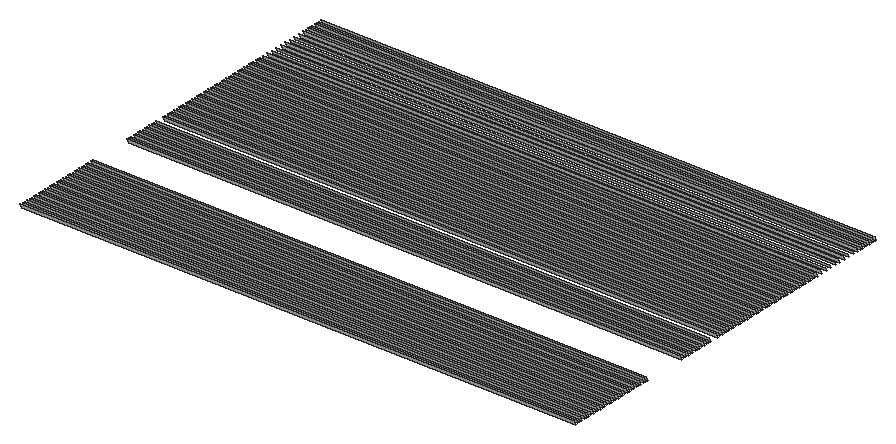
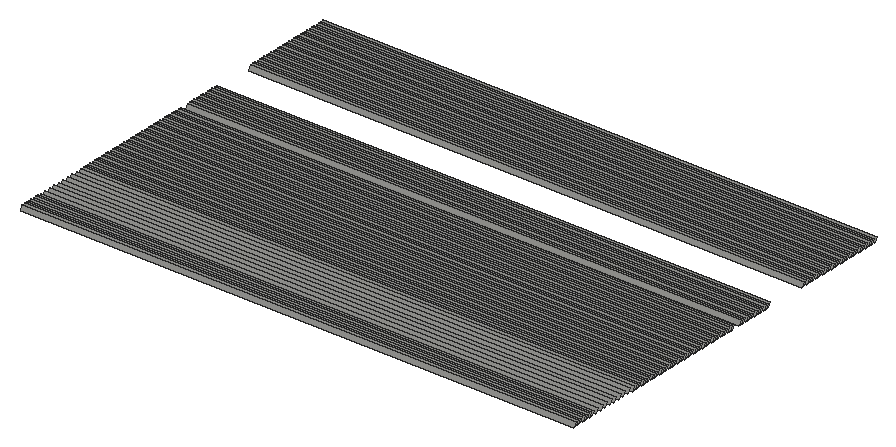
# SketchUp Ruby script. Lengths in inches.
U = 1.inch
M = Sketchup.active_model
def pt(a) = Geom::Point3d.new(a.map { |v| v * U })
def face(e, loops, mat)
  f = e.add_face(loops[0].map { |a| pt(a) })
  loops[1..].each { |l| e.add_face(l.map { |a| pt(a) }).erase! }
  f.material = f.back_material = mat if mat
  f
end
# faces: each face lists its corners as indices into pts; further lists are holes
def faces(e, pts, list, mat = nil) = list.each { |f| face(e, (f[0].is_a?(Array) ? f : [f]).map { |l| l.map { |i| pts[i] } }, mat) }
# xy, xz, yz: faces in a plane at the given z, y or x. An outline is a flat list of corners, or four numbers for a rectangle; further outlines are holes
def ring(l) = l.size == 4 ? [[l[0], l[1]], [l[2], l[1]], [l[2], l[3]], [l[0], l[3]]] : l.each_slice(2).to_a
def flat(e, list, mat, &to3) = list.each { |f| face(e, (f[0].is_a?(Array) ? f : [f]).map { |l| ring(l).map { |u, v| to3.(u, v) } }, mat) }
def xy(e, z, list, mat = nil) = flat(e, list, mat) { |x, y| [x, y, z] }
def xz(e, y, list, mat = nil) = flat(e, list, mat) { |x, z| [x, y, z] }
def yz(e, x, list, mat = nil) = flat(e, list, mat) { |y, z| [x, y, z] }
def lines(e, pts, list) = list.each { |a, b| e.add_line(pt(pts[a]), pt(pts[b])) }
# prism: a flat outline (further loops are holes) pulled along v
def prism(e, loops, v, mat = nil)
  f = face(e, loops, mat); d = Geom::Vector3d.new(v.map { |x| x * U })
  f.pushpull(f.normal.samedirection?(d) ? d.length : -d.length)
end
def box(e, o, s, mat = nil) = prism(e, [[o, [o[0] + s[0], o[1], o[2]], [o[0] + s[0], o[1] + s[1], o[2]], [o[0], o[1] + s[1], o[2]]]], [0, 0, s[2]], mat)
def at(x, y, z, deg = 0) = Geom::Transformation.translation(pt([x, y, z])) * Geom::Transformation.rotation(ORIGIN, Z_AXIS, deg.degrees)
def axes(o, x, y, z) = Geom::Transformation.new([*x, 0, *y, 0, *z, 0, *pt(o).to_a, 1])
def part(name) = M.definitions.add(name)
# library, detail: a bought-in or finely detailed component or shape, given as its bounding box
def library(name, o, s) = part(name).tap { |d| box(d.entities, o, s) }
def detail(e, o, s) = box(e.add_group.entities, o, s)
def put(e, d, t, mat = nil) = e.add_instance(d, t).tap { |i| i.material = mat if mat }
def group(e, t, mat = nil) = e.add_group.tap { |g| g.transformation = t; g.material = mat if mat }.entities
root = M.entities
c1 = part("Group318\#1")
p = [[385.16,196.89,0],[-385.16,196.89,0],[-385.16,193.5,5.875],[385.16,193.5,5.875]]
faces(c1.entities,p,[[0,1,2,3]])
c2 = part("Group319\#1")
p = [[385.16,200.83,0],[-385.16,200.83,0],[-385.16,197.4375,5.875],[385.16,197.4375,5.875]]
faces(c2.entities,p,[[0,1,2,3]])
c3 = part("Group320\#1")
p = [[385.16,204.77,0],[-385.16,204.77,0],[-385.16,201.375,5.875],[385.16,201.375,5.875]]
faces(c3.entities,p,[[0,1,2,3]])
c4 = part("Group321\#1")
p = [[385.16,208.7,0],[-385.16,208.7,0],[-385.16,205.3125,5.875],[385.16,205.3125,5.875]]
faces(c4.entities,p,[[0,1,2,3]])
c5 = part("Group322\#1")
p = [[385.16,212.64,0],[-385.16,212.64,0],[-385.16,209.25,5.875],[385.16,209.25,5.875]]
faces(c5.entities,p,[[0,1,2,3]])
c6 = part("Group323\#1")
p = [[-385.16,213.1875,5.875],[385.16,213.1875,5.875],[385.16,216.58,0],[-385.16,216.58,0]]
faces(c6.entities,p,[[0,1,2,3]])
c7 = part("Group324\#1")
p = [[385.16,220.52,0],[-385.16,220.52,0],[-385.16,217.125,5.875],[385.16,217.125,5.875]]
faces(c7.entities,p,[[0,1,2,3]])
c8 = part("Group325\#1")
p = [[-385.16,221.0625,5.875],[385.16,221.0625,5.875],[385.16,224.45,0],[-385.16,224.45,0]]
faces(c8.entities,p,[[0,1,2,3]])
c9 = part("Group326\#1")
p = [[385.16,228.39,0],[-385.16,228.39,0],[-385.16,225,5.875],[385.16,225,5.875]]
faces(c9.entities,p,[[0,1,2,3]])
c10 = part("Group327\#1")
p = [[-385.16,228.9375,5.875],[385.16,228.9375,5.875],[385.16,232.33,0],[-385.16,232.33,0]]
faces(c10.entities,p,[[0,1,2,3]])
c11 = part("Group328\#1")
p = [[-385.16,232.875,5.875],[385.16,232.875,5.875],[385.16,236.27,0],[-385.16,236.27,0]]
faces(c11.entities,p,[[0,1,2,3]])
c12 = part("Group329\#1")
p = [[385.16,240.2,0],[-385.16,240.2,0],[-385.16,236.8125,5.875],[385.16,236.8125,5.875]]
faces(c12.entities,p,[[0,1,2,3]])
c13 = part("Group330\#1")
p = [[-385.16,240.75,5.875],[385.16,240.75,5.875],[385.16,244.14,0],[-385.16,244.14,0]]
faces(c13.entities,p,[[0,1,2,3]])
c14 = part("Group331\#1")
p = [[-385.16,244.6875,5.875],[385.16,244.6875,5.875],[385.16,248.08,0],[-385.16,248.08,0]]
faces(c14.entities,p,[[0,1,2,3]])
c15 = part("Group332\#1")
p = [[-385.16,248.625,5.875],[385.16,248.625,5.875],[385.16,252.02,0],[-385.16,252.02,0]]
faces(c15.entities,p,[[0,1,2,3]])
c16 = part("Group333\#1")
p = [[385.16,255.95,0],[-385.16,255.95,0],[-385.16,252.5625,5.875],[385.16,252.5625,5.875]]
faces(c16.entities,p,[[0,1,2,3]])
c17 = part("Group334\#1")
p = [[-385.16,256.5,5.875],[385.16,256.5,5.875],[385.16,259.89,0],[-385.16,259.89,0]]
faces(c17.entities,p,[[0,1,2,3]])
c18 = part("Group335\#1")
p = [[-385.16,260.4375,5.875],[385.16,260.4375,5.875],[385.16,263.83,0],[-385.16,263.83,0]]
faces(c18.entities,p,[[0,1,2,3]])
c19 = part("Group336\#1")
p = [[-385.16,264.375,5.875],[385.16,264.375,5.875],[385.16,267.77,0],[-385.16,267.77,0]]
faces(c19.entities,p,[[0,1,2,3]])
c20 = part("Group337\#1")
p = [[385.16,271.7,0],[-385.16,271.7,0],[-385.16,268.3125,5.875],[385.16,268.3125,5.875]]
faces(c20.entities,p,[[0,1,2,3]])
c21 = part("Group338\#1")
p = [[-385.16,272.25,5.875],[385.16,272.25,5.875],[385.16,275.64,0],[-385.16,275.64,0]]
faces(c21.entities,p,[[0,1,2,3]])
c22 = part("Group339\#1")
p = [[385.16,279.58,0],[-385.16,279.58,0],[-385.16,276.1875,5.875],[385.16,276.1875,5.875]]
faces(c22.entities,p,[[0,1,2,3]])
c23 = part("Group340\#1")
p = [[385.16,283.52,0],[-385.16,283.52,0],[-385.16,280.125,5.875],[385.16,280.125,5.875]]
faces(c23.entities,p,[[0,1,2,3]])
c24 = part("Group341\#1")
p = [[385.16,287.45,0],[-385.16,287.45,0],[-385.16,284.0625,5.875],[385.16,284.0625,5.875]]
faces(c24.entities,p,[[0,1,2,3]])
c25 = part("Group342\#1")
p = [[-385.16,288,5.875],[385.16,288,5.875],[385.16,291.39,0],[-385.16,291.39,0]]
faces(c25.entities,p,[[0,1,2,3]])
c26 = part("Group343\#1")
p = [[-385.16,291.9375,5.875],[385.16,291.9375,5.875],[385.16,295.33,0],[-385.16,295.33,0]]
faces(c26.entities,p,[[0,1,2,3]])
c27 = part("Group344\#1")
p = [[385.16,299.27,0],[-385.16,299.27,0],[-385.16,295.875,5.875],[385.16,295.875,5.875]]
faces(c27.entities,p,[[0,1,2,3]])
c28 = part("Group345\#1")
p = [[385.16,303.2,0],[-385.16,303.2,0],[-385.16,299.8125,5.875],[385.16,299.8125,5.875]]
faces(c28.entities,p,[[0,1,2,3]])
c29 = part("Group346\#1")
p = [[385.16,307.14,0],[-385.16,307.14,0],[-385.16,303.75,5.875],[385.16,303.75,5.875]]
faces(c29.entities,p,[[0,1,2,3]])
c30 = part("Group347\#1")
p = [[-385.16,307.6875,5.875],[385.16,307.6875,5.875],[385.16,311.08,0],[-385.16,311.08,0]]
faces(c30.entities,p,[[0,1,2,3]])
c31 = part("Group348\#1")
p = [[-385.16,311.625,5.875],[385.16,311.625,5.875],[385.16,315.02,0],[-385.16,315.02,0]]
faces(c31.entities,p,[[0,1,2,3]])
c32 = part("Group349\#1")
p = [[-385.16,315.5625,5.875],[385.16,315.5625,5.875],[385.16,318.95,0],[-385.16,318.95,0]]
faces(c32.entities,p,[[0,1,2,3]])
c33 = part("Group350\#1")
p = [[-385.16,319.5,5.875],[385.16,319.5,5.875],[385.16,322.89,0],[-385.16,322.89,0]]
faces(c33.entities,p,[[0,1,2,3]])
c34 = part("Group365\#1")
p = [[-385.16,378.5625,5.875],[385.16,378.5625,5.875],[385.16,381.95,0],[-385.16,381.95,0]]
faces(c34.entities,p,[[0,1,2,3]])
c35 = part("Group366\#1")
p = [[385.16,385.89,0],[-385.16,385.89,0],[-385.16,382.5,5.875],[385.16,382.5,5.875]]
faces(c35.entities,p,[[0,1,2,3]])
c36 = part("Group367\#1")
p = [[385.16,389.83,0],[-385.16,389.83,0],[-385.16,386.4375,5.875],[385.16,386.4375,5.875]]
faces(c36.entities,p,[[0,1,2,3]])
c37 = part("Group368\#1")
p = [[385.16,393.77,0],[-385.16,393.77,0],[-385.16,390.375,5.875],[385.16,390.375,5.875]]
faces(c37.entities,p,[[0,1,2,3]])
c38 = part("Group369\#1")
p = [[-385.16,394.3125,5.875],[385.16,394.3125,5.875],[385.16,397.7,0],[-385.16,397.7,0]]
faces(c38.entities,p,[[0,1,2,3]])
c39 = part("Group370\#1")
p = [[-385.16,398.25,5.875],[385.16,398.25,5.875],[385.16,401.64,0],[-385.16,401.64,0]]
faces(c39.entities,p,[[0,1,2,3]])
c40 = part("Group371\#1")
p = [[-385.16,402.1875,5.875],[385.16,402.1875,5.875],[385.16,405.58,0],[-385.16,405.58,0]]
faces(c40.entities,p,[[0,1,2,3]])
c41 = part("Group372\#1")
p = [[-385.16,406.125,5.875],[385.16,406.125,5.875],[385.16,409.52,0],[-385.16,409.52,0]]
faces(c41.entities,p,[[0,1,2,3]])
c42 = part("Group373\#1")
p = [[-385.16,410.0625,5.875],[385.16,410.0625,5.875],[385.16,413.45,0],[-385.16,413.45,0]]
faces(c42.entities,p,[[0,1,2,3]])
c43 = part("Group374\#1")
p = [[385.16,417.39,0],[-385.16,417.39,0],[-385.16,414,5.875],[385.16,414,5.875]]
faces(c43.entities,p,[[0,1,2,3]])
c44 = part("Group375\#1")
p = [[-385.16,417.9375,5.875],[385.16,417.9375,5.875],[385.16,421.33,0],[-385.16,421.33,0]]
faces(c44.entities,p,[[0,1,2,3]])
c45 = part("Group376\#1")
p = [[-385.16,421.875,5.875],[385.16,421.875,5.875],[385.16,425.27,0],[-385.16,425.27,0]]
faces(c45.entities,p,[[0,1,2,3]])
c46 = part("Group377\#1")
p = [[-385.16,425.8125,5.875],[385.16,425.8125,5.875],[385.16,429.2,0],[-385.16,429.2,0]]
faces(c46.entities,p,[[0,1,2,3]])
c47 = part("Group378\#1")
p = [[-385.16,429.75,5.875],[385.16,429.75,5.875],[385.16,433.14,0],[-385.16,433.14,0]]
faces(c47.entities,p,[[0,1,2,3]])
c48 = part("Group381\#1")
p = [[385.16,444.95,0],[-385.16,444.95,0],[-385.16,441.5625,5.875],[385.16,441.5625,5.875]]
faces(c48.entities,p,[[0,1,2,3]])
c49 = part("Group382\#1")
p = [[-385.16,445.5,5.875],[385.16,445.5,5.875],[385.16,448.89,0],[-385.16,448.89,0]]
faces(c49.entities,p,[[0,1,2,3]])
c50 = part("Group383\#1")
p = [[-385.16,449.4375,5.875],[385.16,449.4375,5.875],[385.16,452.83,0],[-385.16,452.83,0]]
faces(c50.entities,p,[[0,1,2,3]])
c51 = part("Group384\#1")
p = [[385.16,456.77,0],[-385.16,456.77,0],[-385.16,453.375,5.875],[385.16,453.375,5.875]]
faces(c51.entities,p,[[0,1,2,3]])
c52 = part("Group385\#1")
p = [[-385.16,457.3125,5.875],[385.16,457.3125,5.875],[385.16,460.7,0],[-385.16,460.7,0]]
faces(c52.entities,p,[[0,1,2,3]])
c53 = part("Group386\#1")
p = [[385.16,464.64,0],[-385.16,464.64,0],[-385.16,461.25,5.875],[385.16,461.25,5.875]]
faces(c53.entities,p,[[0,1,2,3]])
c54 = part("Group387\#1")
p = [[-385.16,465.1875,5.875],[385.16,465.1875,5.875],[385.16,468.58,0],[-385.16,468.58,0]]
faces(c54.entities,p,[[0,1,2,3]])
c55 = part("Group388\#1")
p = [[385.16,472.52,0],[-385.16,472.52,0],[-385.16,469.125,5.875],[385.16,469.125,5.875]]
faces(c55.entities,p,[[0,1,2,3]])
c56 = part("Group389\#1")
p = [[385.16,476.45,0],[-385.16,476.45,0],[-385.16,473.0625,5.875],[385.16,473.0625,5.875]]
faces(c56.entities,p,[[0,1,2,3]])
c57 = part("Group390\#1")
p = [[385.16,480.39,0],[-385.16,480.39,0],[-385.16,477,5.875],[385.16,477,5.875]]
faces(c57.entities,p,[[0,1,2,3]])
c58 = part("Group391\#1")
p = [[385.16,484.33,0],[-385.16,484.33,0],[-385.16,480.9375,5.875],[385.16,480.9375,5.875]]
faces(c58.entities,p,[[0,1,2,3]])
c59 = part("Group392\#1")
p = [[-385.16,484.875,5.875],[385.16,484.875,5.875],[385.16,488.27,0],[-385.16,488.27,0]]
faces(c59.entities,p,[[0,1,2,3]])
c60 = part("Group393\#1")
p = [[-385.16,488.8125,5.875],[385.16,488.8125,5.875],[385.16,492.2,0],[-385.16,492.2,0]]
faces(c60.entities,p,[[0,1,2,3]])
c61 = part("Group394\#1")
p = [[385.16,496.14,0],[-385.16,496.14,0],[-385.16,492.75,5.875],[385.16,492.75,5.875]]
faces(c61.entities,p,[[0,1,2,3]])
c62 = part("Group395\#1")
p = [[-385.16,496.6875,5.875],[385.16,496.6875,5.875],[385.16,500.08,0],[-385.16,500.08,0]]
faces(c62.entities,p,[[0,1,2,3]])
c63 = part("Group396\#1")
p = [[-385.16,500.625,5.875],[385.16,500.625,5.875],[385.16,504.02,0],[-385.16,504.02,0]]
faces(c63.entities,p,[[0,1,2,3]])
c64 = part("Group397\#1")
p = [[-385.16,504.5625,5.875],[385.16,504.5625,5.875],[385.16,507.95,0],[-385.16,507.95,0]]
faces(c64.entities,p,[[0,1,2,3]])
c65 = part("Group398\#1")
p = [[-385.16,508.5,5.875],[385.16,508.5,5.875],[385.16,511.89,0],[-385.16,511.89,0]]
faces(c65.entities,p,[[0,1,2,3]])
c66 = part("Group399\#1")
p = [[-385.16,512.4375,5.875],[385.16,512.4375,5.875],[385.16,515.83,0],[-385.16,515.83,0]]
faces(c66.entities,p,[[0,1,2,3]])
c67 = part("Group400\#1")
p = [[385.16,519.77,0],[-385.16,519.77,0],[-385.16,516.375,5.875],[385.16,516.375,5.875]]
faces(c67.entities,p,[[0,1,2,3]])
c68 = part("Group401\#1")
p = [[385.16,523.7,0],[-385.16,523.7,0],[-385.16,520.3125,5.875],[385.16,520.3125,5.875]]
faces(c68.entities,p,[[0,1,2,3]])
c69 = part("Group402\#1")
p = [[-385.16,524.25,5.875],[385.16,524.25,5.875],[385.16,527.64,0],[-385.16,527.64,0]]
faces(c69.entities,p,[[0,1,2,3]])
c70 = part("Group403\#1")
p = [[-385.16,528.1875,5.875],[385.16,528.1875,5.875],[385.16,531.58,0],[-385.16,531.58,0]]
faces(c70.entities,p,[[0,1,2,3]])
c71 = part("Group404\#1")
p = [[385.16,535.52,0],[-385.16,535.52,0],[-385.16,532.125,5.875],[385.16,532.125,5.875]]
faces(c71.entities,p,[[0,1,2,3]])
c72 = part("Group405\#1")
p = [[385.16,539.45,0],[-385.16,539.45,0],[-385.16,536.0625,5.875],[385.16,536.0625,5.875]]
faces(c72.entities,p,[[0,1,2,3]])
c73 = part("Group406\#1")
p = [[-385.16,540,5.875],[385.16,540,5.875],[385.16,543.39,0],[-385.16,543.39,0]]
faces(c73.entities,p,[[0,1,2,3]])
c74 = part("Group407\#1")
p = [[385.16,547.33,0],[-385.16,547.33,0],[-385.16,543.9375,5.875],[385.16,543.9375,5.875]]
faces(c74.entities,p,[[0,1,2,3]])
c75 = part("Group408\#1")
p = [[385.16,551.27,0],[-385.16,551.27,0],[-385.16,547.875,5.875],[385.16,547.875,5.875]]
faces(c75.entities,p,[[0,1,2,3]])
c76 = part("Group409\#1")
p = [[-385.16,551.8125,5.875],[385.16,551.8125,5.875],[385.16,555.2,0],[-385.16,555.2,0]]
faces(c76.entities,p,[[0,1,2,3]])
c77 = part("Group410\#1")
p = [[-385.16,555.75,5.875],[385.16,555.75,5.875],[385.16,559.14,0],[-385.16,559.14,0]]
faces(c77.entities,p,[[0,1,2,3]])
c78 = part("Group411\#1")
p = [[385.16,563.08,0],[-385.16,563.08,0],[-385.16,559.6875,5.875],[385.16,559.6875,5.875]]
faces(c78.entities,p,[[0,1,2,3]])
c79 = part("Group412\#1")
p = [[-385.16,563.625,5.875],[385.16,563.625,5.875],[385.16,567.02,0],[-385.16,567.02,0]]
faces(c79.entities,p,[[0,1,2,3]])
c80 = part("Group413\#1")
p = [[385.16,570.95,0],[-385.16,570.95,0],[-385.16,567.5625,5.875],[385.16,567.5625,5.875]]
faces(c80.entities,p,[[0,1,2,3]])
c81 = part("Group414\#1")
p = [[385.16,574.89,0],[-385.16,574.89,0],[-385.16,571.5,5.875],[385.16,571.5,5.875]]
faces(c81.entities,p,[[0,1,2,3]])
c82 = part("Group415\#1")
p = [[385.16,578.83,0],[-385.16,578.83,0],[-385.16,575.4375,5.875],[385.16,575.4375,5.875]]
faces(c82.entities,p,[[0,1,2,3]])
c83 = part("Group416\#1")
p = [[-385.16,579.375,5.875],[385.16,579.375,5.875],[385.16,582.77,0],[-385.16,582.77,0]]
faces(c83.entities,p,[[0,1,2,3]])
c84 = part("Group417\#1")
p = [[385.16,586.7,0],[-385.16,586.7,0],[-385.16,583.3125,5.875],[385.16,583.3125,5.875]]
faces(c84.entities,p,[[0,1,2,3]])
c85 = part("Group418\#1")
p = [[385.16,590.64,0],[-385.16,590.64,0],[-385.16,587.25,5.875],[385.16,587.25,5.875]]
faces(c85.entities,p,[[0,1,2,3]])
c86 = part("Group419\#1")
p = [[385.16,594.58,0],[-385.16,594.58,0],[-385.16,591.1875,5.875],[385.16,591.1875,5.875]]
faces(c86.entities,p,[[0,1,2,3]])
c87 = part("Group420\#1")
p = [[-385.16,595.125,5.875],[385.16,595.125,5.875],[385.16,598.52,0],[-385.16,598.52,0]]
faces(c87.entities,p,[[0,1,2,3]])
c88 = part("Group421\#1")
p = [[385.16,602.45,0],[-385.16,602.45,0],[-385.16,599.0625,5.875],[385.16,599.0625,5.875]]
faces(c88.entities,p,[[0,1,2,3]])
c89 = part("Group422\#1")
p = [[385.16,606.39,0],[-385.16,606.39,0],[-385.16,603,5.875],[385.16,603,5.875]]
faces(c89.entities,p,[[0,1,2,3]])
c90 = part("Group423\#1")
p = [[-385.16,606.9375,5.875],[385.16,606.9375,5.875],[385.16,610.33,0],[-385.16,610.33,0]]
faces(c90.entities,p,[[0,1,2,3]])
c91 = part("Group424\#1")
p = [[-385.16,610.875,5.875],[385.16,610.875,5.875],[385.16,614.27,0],[-385.16,614.27,0]]
faces(c91.entities,p,[[0,1,2,3]])
c92 = part("Group425\#1")
p = [[-385.16,614.8125,5.875],[385.16,614.8125,5.875],[385.16,618.2,0],[-385.16,618.2,0]]
faces(c92.entities,p,[[0,1,2,3]])
c93 = part("Group427\#1")
p = [[385.16,626.08,0],[-385.16,626.08,0],[-385.16,622.6875,5.875],[385.16,622.6875,5.875]]
faces(c93.entities,p,[[0,1,2,3]])
c94 = part("Group429\#1")
p = [[-385.16,630.5625,5.875],[385.16,630.5625,5.875],[385.16,633.95,0],[-385.16,633.95,0]]
faces(c94.entities,p,[[0,1,2,3]])
c95 = part("Group431\#1")
p = [[-385.16,638.4375,5.875],[385.16,638.4375,5.875],[385.16,641.83,0],[-385.16,641.83,0]]
faces(c95.entities,p,[[0,1,2,3]])
c96 = part("Group433\#1")
p = [[-385.16,646.3125,5.875],[385.16,646.3125,5.875],[385.16,649.7,0],[-385.16,649.7,0]]
faces(c96.entities,p,[[0,1,2,3]])
c97 = part("Group435\#1")
p = [[-385.16,654.1875,5.875],[385.16,654.1875,5.875],[385.16,657.58,0],[-385.16,657.58,0]]
faces(c97.entities,p,[[0,1,2,3]])
c98 = part("Group437\#1")
p = [[385.16,665.45,0],[-385.16,665.45,0],[-385.16,662.0625,5.875],[385.16,662.0625,5.875]]
faces(c98.entities,p,[[0,1,2,3]])
c99 = part("Group439\#1")
p = [[385.16,673.33,0],[-385.16,673.33,0],[-385.16,669.9375,5.875],[385.16,669.9375,5.875]]
faces(c99.entities,p,[[0,1,2,3]])
c100 = part("Group441\#1")
p = [[-385.16,677.8125,5.875],[385.16,677.8125,5.875],[385.16,681.2,0],[-385.16,681.2,0]]
faces(c100.entities,p,[[0,1,2,3]])
c101 = part("Group443\#1")
p = [[-385.16,685.6875,5.875],[385.16,685.6875,5.875],[385.16,689.08,0],[-385.16,689.08,0]]
faces(c101.entities,p,[[0,1,2,3]])
c102 = part("Group444\#1")
p = [[-385.16,689.625,5.875],[385.16,689.625,5.875],[385.16,693.02,0],[-385.16,693.02,0]]
faces(c102.entities,p,[[0,1,2,3]])
c103 = part("Group445\#1")
p = [[-385.16,693.5625,5.875],[385.16,693.5625,5.875],[385.16,696.95,0],[-385.16,696.95,0]]
faces(c103.entities,p,[[0,1,2,3]])
c104 = part("Group446\#1")
p = [[-385.16,697.5,5.875],[385.16,697.5,5.875],[385.16,700.89,0],[-385.16,700.89,0]]
faces(c104.entities,p,[[0,1,2,3]])
c105 = part("Group447\#1")
p = [[-385.16,701.4375,5.875],[385.16,701.4375,5.875],[385.16,704.83,0],[-385.16,704.83,0]]
faces(c105.entities,p,[[0,1,2,3]])
c106 = part("Group448\#1")
p = [[-385.16,705.375,5.875],[385.16,705.375,5.875],[385.16,708.77,0],[-385.16,708.77,0]]
faces(c106.entities,p,[[0,1,2,3]])
c107 = part("Group449\#1")
p = [[385.16,712.7,0],[-385.16,712.7,0],[-385.16,709.3125,5.875],[385.16,709.3125,5.875]]
faces(c107.entities,p,[[0,1,2,3]])
c108 = part("Group450\#1")
p = [[-385.16,713.25,5.875],[385.16,713.25,5.875],[385.16,716.64,0],[-385.16,716.64,0]]
faces(c108.entities,p,[[0,1,2,3]])
c109 = part("Group451\#1")
p = [[-385.16,717.1875,5.875],[385.16,717.1875,5.875],[385.16,720.58,0],[-385.16,720.58,0]]
faces(c109.entities,p,[[0,1,2,3]])
put(root,c1,at(1937.93,1232.46,154.625))
put(root,c2,at(1937.93,1232.46,154.625))
put(root,c3,at(1937.93,1232.46,154.625))
put(root,c4,at(1937.93,1232.46,154.625))
put(root,c5,at(1937.93,1232.46,154.625))
put(root,c6,at(1937.93,1232.46,154.625))
put(root,c7,at(1937.93,1232.46,154.625))
put(root,c8,at(1937.93,1232.46,154.625))
put(root,c9,at(1937.93,1232.46,154.625))
put(root,c10,at(1937.93,1232.46,154.625))
put(root,c11,at(1937.93,1232.46,154.625))
put(root,c12,at(1937.93,1232.46,154.625))
put(root,c13,at(1937.93,1232.46,154.625))
put(root,c14,at(1937.93,1232.46,154.625))
put(root,c15,at(1937.93,1232.46,154.625))
put(root,c16,at(1937.93,1232.46,154.625))
put(root,c17,at(1937.93,1232.46,154.625))
put(root,c18,at(1937.93,1232.46,154.625))
put(root,c19,at(1937.93,1232.46,154.625))
put(root,c20,at(1937.93,1232.46,154.625))
put(root,c21,at(1937.93,1232.46,154.625))
put(root,c22,at(1937.93,1232.46,154.625))
put(root,c23,at(1937.93,1232.46,154.625))
put(root,c24,at(1937.93,1232.46,154.625))
put(root,c25,at(1937.93,1232.46,154.625))
put(root,c26,at(1937.93,1232.46,154.625))
put(root,c27,at(1937.93,1232.46,154.625))
put(root,c28,at(1937.93,1232.46,154.625))
put(root,c29,at(1937.93,1232.46,154.625))
put(root,c30,at(1937.93,1232.46,154.625))
put(root,c31,at(1937.93,1232.46,154.625))
put(root,c32,at(1937.93,1232.46,154.625))
put(root,c33,at(1937.93,1232.46,154.625))
put(root,c34,at(1937.93,1232.46,154.625))
put(root,c35,at(1937.93,1232.46,154.625))
put(root,c36,at(1937.93,1232.46,154.625))
put(root,c37,at(1937.93,1232.46,154.625))
put(root,c38,at(1937.93,1232.46,154.625))
put(root,c39,at(1937.93,1232.46,154.625))
put(root,c40,at(1937.93,1232.46,154.625))
put(root,c41,at(1937.93,1232.46,154.625))
put(root,c42,at(1937.93,1232.46,154.625))
put(root,c43,at(1937.93,1232.46,154.625))
put(root,c44,at(1937.93,1232.46,154.625))
put(root,c45,at(1937.93,1232.46,154.625))
put(root,c46,at(1937.93,1232.46,154.625))
put(root,c47,at(1937.93,1232.46,154.625))
put(root,c48,at(1937.93,1232.46,154.625))
put(root,c49,at(1937.93,1232.46,154.625))
put(root,c50,at(1937.93,1232.46,154.625))
put(root,c51,at(1937.93,1232.46,154.625))
put(root,c52,at(1937.93,1232.46,154.625))
put(root,c53,at(1937.93,1232.46,154.625))
put(root,c54,at(1937.93,1232.46,154.625))
put(root,c55,at(1937.93,1232.46,154.625))
put(root,c56,at(1937.93,1232.46,154.625))
put(root,c57,at(1937.93,1232.46,154.625))
put(root,c58,at(1937.93,1232.46,154.625))
put(root,c59,at(1937.93,1232.46,154.625))
put(root,c60,at(1937.93,1232.46,154.625))
put(root,c61,at(1937.93,1232.46,154.625))
put(root,c62,at(1937.93,1232.46,154.625))
put(root,c63,at(1937.93,1232.46,154.625))
put(root,c64,at(1937.93,1232.46,154.625))
put(root,c65,at(1937.93,1232.46,154.625))
put(root,c66,at(1937.93,1232.46,154.625))
put(root,c67,at(1937.93,1232.46,154.625))
put(root,c68,at(1937.93,1232.46,154.625))
put(root,c69,at(1937.93,1232.46,154.625))
put(root,c70,at(1937.93,1232.46,154.625))
put(root,c71,at(1937.93,1232.46,154.625))
put(root,c72,at(1937.93,1232.46,154.625))
put(root,c73,at(1937.93,1232.46,154.625))
put(root,c74,at(1937.93,1232.46,154.625))
put(root,c75,at(1937.93,1232.46,154.625))
put(root,c76,at(1937.93,1232.46,154.625))
put(root,c77,at(1937.93,1232.46,154.625))
put(root,c78,at(1937.93,1232.46,154.625))
put(root,c79,at(1937.93,1232.46,154.625))
put(root,c80,at(1937.93,1232.46,154.625))
put(root,c81,at(1937.93,1232.46,154.625))
put(root,c82,at(1937.93,1232.46,154.625))
put(root,c83,at(1937.93,1232.46,154.625))
put(root,c84,at(1937.93,1232.46,154.625))
put(root,c85,at(1937.93,1232.46,154.625))
put(root,c86,at(1937.93,1232.46,154.625))
put(root,c87,at(1937.93,1232.46,154.625))
put(root,c88,at(1937.93,1232.46,154.625))
put(root,c89,at(1937.93,1232.46,154.625))
put(root,c90,at(1937.93,1232.46,154.625))
put(root,c91,at(1937.93,1232.46,154.625))
put(root,c92,at(1937.93,1232.46,154.625))
put(root,c93,at(1937.93,1232.46,154.625))
put(root,c94,at(1937.93,1232.46,154.625))
put(root,c95,at(1937.93,1232.46,154.625))
put(root,c96,at(1937.93,1232.46,154.625))
put(root,c97,at(1937.93,1232.46,154.625))
put(root,c98,at(1937.93,1232.46,154.625))
put(root,c99,at(1937.93,1232.46,154.625))
put(root,c100,at(1937.93,1232.46,154.625))
put(root,c101,at(1937.93,1232.46,154.625))
put(root,c102,at(1937.93,1232.46,154.625))
put(root,c103,at(1937.93,1232.46,154.625))
put(root,c104,at(1937.93,1232.46,154.625))
put(root,c105,at(1937.93,1232.46,154.625))
put(root,c106,at(1937.93,1232.46,154.625))
put(root,c107,at(1937.93,1232.46,154.625))
put(root,c108,at(1937.93,1232.46,154.625))
put(root,c109,at(1937.93,1232.46,154.625))
